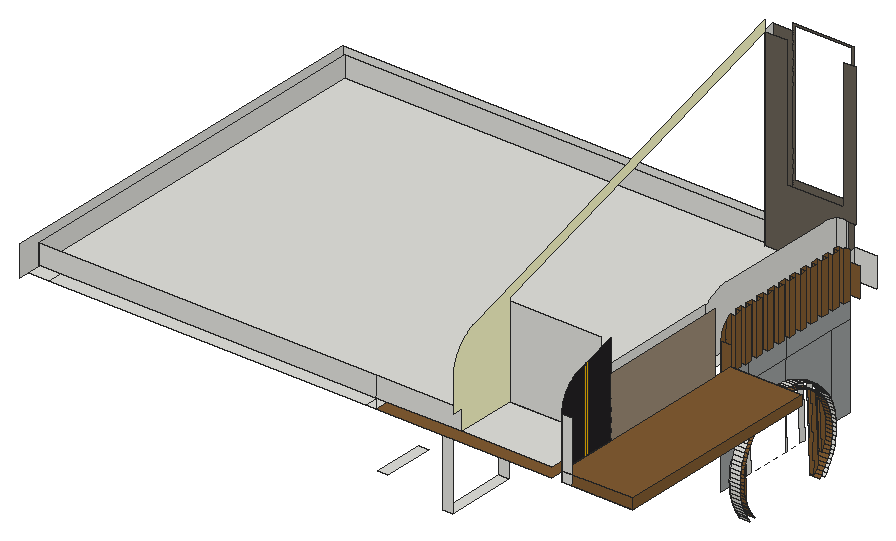
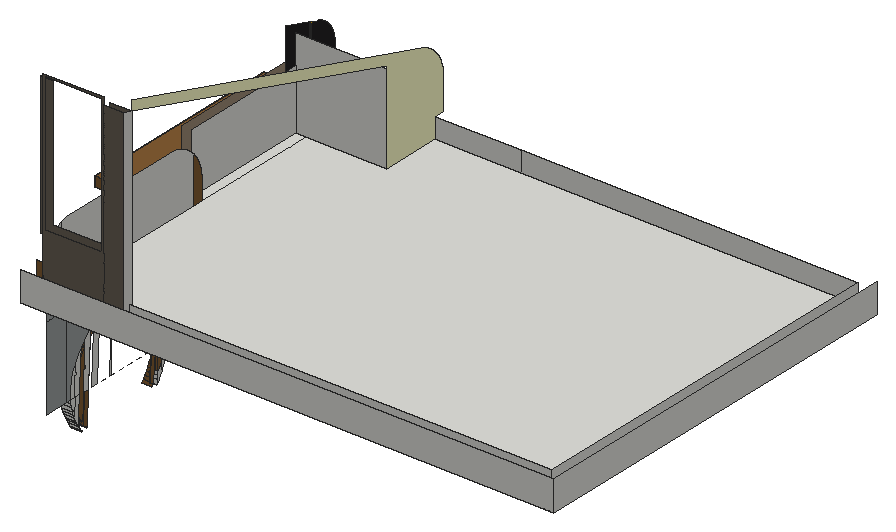
# SketchUp Ruby script. Lengths in inches.
U = 1.inch
M = Sketchup.active_model
def pt(a) = Geom::Point3d.new(a.map { |v| v * U })
def face(e, loops, mat)
  f = e.add_face(loops[0].map { |a| pt(a) })
  loops[1..].each { |l| e.add_face(l.map { |a| pt(a) }).erase! }
  f.material = f.back_material = mat if mat
  f
end
# faces: each face lists its corners as indices into pts; further lists are holes
def faces(e, pts, list, mat = nil) = list.each { |f| face(e, (f[0].is_a?(Array) ? f : [f]).map { |l| l.map { |i| pts[i] } }, mat) }
# xy, xz, yz: faces in a plane at the given z, y or x. An outline is a flat list of corners, or four numbers for a rectangle; further outlines are holes
def ring(l) = l.size == 4 ? [[l[0], l[1]], [l[2], l[1]], [l[2], l[3]], [l[0], l[3]]] : l.each_slice(2).to_a
def flat(e, list, mat, &to3) = list.each { |f| face(e, (f[0].is_a?(Array) ? f : [f]).map { |l| ring(l).map { |u, v| to3.(u, v) } }, mat) }
def xy(e, z, list, mat = nil) = flat(e, list, mat) { |x, y| [x, y, z] }
def xz(e, y, list, mat = nil) = flat(e, list, mat) { |x, z| [x, y, z] }
def yz(e, x, list, mat = nil) = flat(e, list, mat) { |y, z| [x, y, z] }
def lines(e, pts, list) = list.each { |a, b| e.add_line(pt(pts[a]), pt(pts[b])) }
# prism: a flat outline (further loops are holes) pulled along v
def prism(e, loops, v, mat = nil)
  f = face(e, loops, mat); d = Geom::Vector3d.new(v.map { |x| x * U })
  f.pushpull(f.normal.samedirection?(d) ? d.length : -d.length)
end
def box(e, o, s, mat = nil) = prism(e, [[o, [o[0] + s[0], o[1], o[2]], [o[0] + s[0], o[1] + s[1], o[2]], [o[0], o[1] + s[1], o[2]]]], [0, 0, s[2]], mat)
def at(x, y, z, deg = 0) = Geom::Transformation.translation(pt([x, y, z])) * Geom::Transformation.rotation(ORIGIN, Z_AXIS, deg.degrees)
def axes(o, x, y, z) = Geom::Transformation.new([*x, 0, *y, 0, *z, 0, *pt(o).to_a, 1])
def part(name) = M.definitions.add(name)
# library, detail: a bought-in or finely detailed component or shape, given as its bounding box
def library(name, o, s) = part(name).tap { |d| box(d.entities, o, s) }
def detail(e, o, s) = box(e.add_group.entities, o, s)
def put(e, d, t, mat = nil) = e.add_instance(d, t).tap { |i| i.material = mat if mat }
def group(e, t, mat = nil) = e.add_group.tap { |g| g.transformation = t; g.material = mat if mat }.entities
root = M.entities
M.materials.add("C08_Toffee_Ember").color = [130, 92, 50]
M.materials.add("D05_Goldenrod_Hue").color = [255, 191, 0]
M.materials.add("Denim_03_1K").color = [156, 160, 160]
M.materials.add("E01_Mint_Frost").color = [255, 255, 204]
M.materials.add("Marble_07_1K").color = [36, 34, 36]
M.materials.add("Plaster_02_1K").color = [157, 140, 119]
M.materials.add("Plaster_04_1K").color = [106, 98, 87]
xy(root,297,[[206.67,78,212.67,120]])
xy(root,339,[[206.67,30,212.67,60],[206.67,78,212.67,120]])
xy(root,378,[[5.5,21,17.5,141],[17.5,21,206.67,141],[206.67,21,212.67,141],[212.67,135,311.5,141],[5.5,141,17.5,255],
  [17.5,141,311.5,249],[317.5,154.16,320.5,157.74],[317.5,161.32,320.5,165.4],[317.5,169.49,320.5,173.57],[317.5,177.66,320.5,181.74],
  [317.5,185.82,320.5,189.91],[317.5,193.99,320.5,198.08],[317.5,202.16,320.5,206.24],[317.5,210.33,320.5,214.41],[317.5,218.5,320.5,222.58],
  [317.5,226.66,320.5,230.75],[317.5,234.83,320.5,238.92]])
xy(root,378,[[212.67,21,212.67,135,329.5,135,329.5,147,365.5,147,365.5,21,323.5,21,323.5,57,317.5,57,317.5,21]],"C08_Toffee_Ember")
xy(root,382.3,[[263.5,247,311.5,253]])
xy(root,384,[[11.5,21,263.5,21,263.5,57,311.5,57,311.5,249,11.5,249],[263.5,21,317.5,57],[311.5,57,317.5,135]])
xy(root,384,[[323.5,21,365.5,147]],"C08_Toffee_Ember")
xz(root,21,[[323.5,378,329.5,384],[11.5,384,212.67,396],[212.67,384,263.5,396],[323.5,384,329.5,414]])
xz(root,21,[[329.5,378,365.5,384]],"C08_Toffee_Ember")
xz(root,57,[[263.5,384,317.5,437.47]])
xz(root,78,[[206.67,297,212.67,339]])
xz(root,120,[[206.67,297,212.67,339]])
xz(root,135,[[311.5,384,317.5,396],[317.5,384,323.5,396]])
xz(root,147,[[317.5,378,317.5,396,323.5,396,323.5,384,365.5,384,365.5,378]],"C08_Toffee_Ember")
xz(root,154.16,[[317.5,378,320.5,406.92]],"C08_Toffee_Ember")
xz(root,157.74,[[317.5,378,320.5,407.92]],"C08_Toffee_Ember")
xz(root,161.32,[[317.5,378,320.5,408]],"C08_Toffee_Ember")
xz(root,165.4,[[317.5,378,320.5,408]],"C08_Toffee_Ember")
xz(root,169.49,[[317.5,378,320.5,408]],"C08_Toffee_Ember")
xz(root,173.57,[[317.5,378,320.5,408]],"C08_Toffee_Ember")
xz(root,177.66,[[317.5,378,320.5,408]],"C08_Toffee_Ember")
xz(root,181.74,[[317.5,378,320.5,408]],"C08_Toffee_Ember")
xz(root,185.82,[[317.5,378,320.5,408]],"C08_Toffee_Ember")
xz(root,189.91,[[317.5,378,320.5,408]],"C08_Toffee_Ember")
xz(root,193.99,[[317.5,378,320.5,408]],"C08_Toffee_Ember")
xz(root,198.08,[[317.5,378,320.5,408]],"C08_Toffee_Ember")
xz(root,202.16,[[317.5,378,320.5,408]],"C08_Toffee_Ember")
xz(root,206.24,[[317.5,378,320.5,408]],"C08_Toffee_Ember")
xz(root,210.33,[[317.5,378,320.5,408]],"C08_Toffee_Ember")
xz(root,214.41,[[317.5,378,320.5,408]],"C08_Toffee_Ember")
xz(root,218.5,[[317.5,378,320.5,408]],"C08_Toffee_Ember")
xz(root,222.58,[[317.5,378,320.5,408]],"C08_Toffee_Ember")
xz(root,226.66,[[317.5,378,320.5,408]],"C08_Toffee_Ember")
xz(root,230.75,[[317.5,378,320.5,408]],"C08_Toffee_Ember")
xz(root,234.83,[[317.5,378,320.5,407.41]],"C08_Toffee_Ember")
xz(root,238.92,[[317.5,378,320.5,405.09]],"C08_Toffee_Ember")
xz(root,243,[[317.5,378,323.5,396]],"C08_Toffee_Ember")
xz(root,247,[[263.5,382.3,311.5,382.3,311.5,413.98,317.5,413.98,317.5,498,310.5,498,310.5,421,276.5,421,276.5,498,263.5,498]],"Plaster_04_1K")
xz(root,249,[[11.5,384,311.5,396]])
xz(root,253,[[263.5,382.3,275.5,500.01],[275.5,382.3,275.5,500.01,276.5,500.01,276.5,421,310.5,421,310.5,503,276.5,503,276.5,500.01,275.5,500.01,275.5,504,311.5,504,311.5,382.3]],"Plaster_04_1K")
xz(root,255,[[5.5,378,323.5,396]])
yz(root,5.5,[[15,378,255,396]])
yz(root,11.5,[[21,384,249,396]])
yz(root,263.5,[[247,382.3,247,498.15,253,500.01,253,382.3]])
yz(root,263.5,[[21,384,21,396,15,396,15,415.29,15.02,415.87,15.0625,416.5,15.12,417.12,15.19,417.74,15.28,418.36,15.39,418.97,15.51,419.58,15.65,420.19,15.81,420.8,15.98,421.4,16.16,421.99,16.58,423.17,16.82,423.75,17.07,424.32,17.33,424.89,17.61,425.44,17.9,426,18.21,426.54,18.53,427.07,18.87,427.6,19.22,428.12,19.58,428.625,19.96,429.12,20.35,429.61,20.75,430.09,21,430.37,21.17,430.55,21.59,431.01,22.03,431.45,22.49,431.88,22.61,432,22.95,432.3,23.42,432.71,23.9,433.1,24.4,433.49,24.9,433.85,25.42,434.21,25.9375,434.55,26.47,434.88,27.01,435.19,27.56,435.49,28.12,435.77,28.68,436.04,29.25,436.3,29.83,436.54,30.41,436.76,30.96,436.95,247,504,247,498,57,439.04,57,384]],"E01_Mint_Frost")
yz(root,311.5,[[247,382.3,253,382.3,253,396,249,396,249,384,247,384],[141,384,141,411.58,141.14,411.74,141.65,412.29,142.17,412.83,142.71,413.35,143.26,413.86,143.83,414.35,144.41,414.82,145.01,415.27,145.625,415.7,146.25,416.12,146.89,416.52,147.53,416.89,148.19,417.25,148.86,417.58,149.55,417.9,150.24,418.19,150.93,418.46,151.64,418.71,152.35,418.94,153.08,419.15,153.8,419.34,154.53,419.5,155.27,419.64,156.01,419.76,156.76,419.85,157.5,419.92,158.25,419.97,159,420,231,420,231.76,419.99,232.51,419.96,233.26,419.91,234.01,419.83,234.76,419.73,235.51,419.6,236.25,419.45,236.98,419.28,237.71,419.08,238.4375,418.86,239.15,418.62,239.59,418.46,239.59,384],[239.59,384,239.59,418.46,239.86,418.36,240.56,418.07,241.25,417.76,241.93,417.43,242.6,417.08,243.25,416.71,243.9,416.3125,244.53,415.9,245.15,415.47,245.75,415.01,246.34,414.54,246.92,414.05,247,413.98,247,384],[247,384,249,384,249,411.97,248.54,412.48,248.02,413.02,247.48,413.54,247,413.98]])
yz(root,311.5,[[135,384,135,396,135.03,396.75,135.08,397.5,135.15,398.24,135.24,398.99,135.36,399.73,135.5,400.47,135.66,401.2,135.85,401.92,136.06,402.65,136.29,403.36,136.54,404.07,136.81,404.76,137.1,405.45,137.42,406.14,137.75,406.81,138.11,407.47,138.48,408.11,138.88,408.75,139.3,409.375,139.73,409.99,140.18,410.59,140.65,411.17,141,411.58,141,384]],"C08_Toffee_Ember")
yz(root,317.5,[[160.39,296.18,160.08,302.125,159.9,302.43,158.98,304.29,158.18,306.2,157.5,308.16,156.95,310.15,156.52,312.18,156.22,314.23,156.125,315.33,156.09,315.33,156.78,301.98,157.26,301.01,158.39,299.05,159.64,297.17],[219.71,299.24,220.35,300.3,221.4,302.31,222.32,304.37,222.7,305.375,222.18,315.33,218.88,315.33,219.4,305.1875],[156.78,301.98,156.09,315.33,153.12,315.33,153.24,313.89,153.5625,311.65,154.03,309.44,154.64,307.26,155.38,305.125,156.26,303.04],[222.7,305.375,223.11,306.49,223.77,308.65,224.28,310.86,224.66,313.09,224.9,315.33,222.18,315.33],[153.12,315.33,156.09,315.33,156.04,316.3,155.3,330.625,154.89,329.51,154.23,327.35,153.72,325.14,153.34,322.91,153.1,320.67,153,318.41,153.05,316.14],
  [156.09,315.33,156.125,315.33,156.04,316.3],[159.4,315.33,162.7,315.33,161.62,336.39,161.375,341.07,160.12,339.49,158.82,337.63,158.29,336.76,158.6,330.8125],[166.01,315.33,169.3125,315.33,167.87,343.33,167.68,346.99,166.37,346,164.65,344.52,164.51,344.375,164.72,340.32],[194.92,315.33,195.75,315.33,194.92,331.43],[205.66,315.33,208.96,315.33,207.41,345.37,207.23,349.03,206.7,349.35,204.69,350.4,203.83,350.78,204.01,347.375],
  [212.27,315.33,215.57,315.33,214.35,339.11,214.1,343.79,213.9375,343.96,212.26,345.48,210.65,346.76,210.86,342.71],[218.88,315.33,222.18,315.33,221.96,319.7,221.22,334.02,220.74,334.99,219.61,336.95,218.36,338.83,217.61,339.82,217.92,333.875],[222.18,315.33,224.9,315.33,225,317.59,224.95,319.86,224.76,322.11,224.4375,324.35,223.97,326.56,223.36,328.74,222.62,330.875,221.74,332.96,221.22,334.02,221.96,319.7],[57,384,135,420]])
yz(root,317.5,[[216.38,299.61,216.66,300,217.74,301.78,218.7,303.61,219.4,305.1875,218.88,315.33,217.92,333.875,217.0625,335.37,215.91,337.09,214.66,338.75,214.35,339.11,215.57,315.33],[160.08,302.125,159.4,315.33,158.6,330.8125,158.46,330.49,157.73,328.55,157.13,326.57,156.66,324.55,156.31,322.51,156.09,320.44,156,318.37,156.04,316.3,156.125,315.33,156.22,314.23,156.52,312.18,156.95,310.15,157.5,308.16,158.18,306.2,158.98,304.29,159.9,302.43],[194.92,331.43,194.92,350.45,193.93,350.62],[147,378,150.58,378,150.58,404.46,150.56,404.44,150.3,404.17,149.8,403.61,149.57,403.3125,149.34,403.01,149.12,402.71,148.72,402.07,148.53,401.75,148.35,401.42,148.1875,401.08,148.03,400.74,147.88,400.39,147.75,400.04,147.625,399.6875,147.51,399.33,147.41,398.97,147.32,398.61,147.24,398.24,147.17,397.87,147.11,397.5,147.03,396.75,147.01,396.375,147,396],[150.58,378,154.16,378,154.16,406.92,153.92,406.8125,153.58,406.65,153.25,406.47,152.93,406.28,152.29,405.88,151.99,405.66,151.6875,405.43,151.39,405.2,150.83,404.7,150.58,404.46],
  [157.74,378,161.32,378,161.32,408,159,408,158.625,407.99,158.25,407.97,157.875,407.93,157.74,407.92],[165.4,378,169.49,408],[173.57,378,177.66,408],[181.74,378,185.82,408],[189.91,378,193.99,408],
  [198.08,378,202.16,408],[206.24,378,210.33,408],[214.41,378,218.5,408],[222.58,378,226.66,408],[230.75,378,234.83,378,234.83,407.41,234.72,407.45,234,407.65,233.63,407.74,233.26,407.81,232.88,407.87,232.51,407.92,232.13,407.96,231.76,407.98,231.38,408,230.75,408],
  [238.92,378,243,378,243,396.38,242.98,396.76,242.96,397.13,242.92,397.51,242.87,397.88,242.81,398.26,242.74,398.63,242.65,399,242.45,399.72,242.33,400.08,242.19,400.4375,242.05,400.79,241.9,401.13,241.56,401.81,241.37,402.14,240.97,402.78,240.75,403.09,240.52,403.39,240.29,403.6875,240.04,403.97,239.79,404.25,239.53,404.53,239.25,404.79,238.97,405.04,238.92,405.09]],"C08_Toffee_Ember")
yz(root,317.5,[[147,315.33,153.12,315.33,153.05,316.14,153,318.41,153.1,320.67,153.34,322.91,153.72,325.14,154.23,327.35,154.89,329.51,155.3,330.625,155.68,331.63,156.6,333.69,157.65,335.7,158.29,336.76,158.82,337.63,160.12,339.49,161.375,341.07,161.52,341.26,163.04,342.9375,164.51,344.375,164.65,344.52,166.37,346,167.68,346.99,167.68,365.07,147,365.07],[224.9,315.33,228.75,315.33,228.75,365.07,194.92,365.07,194.92,353.49,196.14,353.28,198.35,352.77,200.51,352.11,202.63,351.32,203.83,350.78,204.69,350.4,206.7,349.35,207.23,349.03,208.63,348.18,210.49,346.88,210.65,346.76,212.26,345.48,213.9375,343.96,214.1,343.79,215.52,342.35,217,340.63,217.61,339.82,218.36,338.83,219.61,336.95,220.74,334.99,221.22,334.02,221.74,332.96,222.62,330.875,223.36,328.74,223.97,326.56,224.4375,324.35,224.76,322.11,224.95,319.86,225,317.59],[228.75,315.33,243,365.07],[167.68,346.99,168.17,347.36,170.05,348.61,170.875,349.08,172.01,349.74,174.04,350.74,176.125,351.62,178.26,352.36,180.44,352.97,182.65,353.4375,184.89,353.76,187.14,353.95,189.41,354,191.67,353.9,193.91,353.66,194.92,353.49,194.92,365.07,167.68,365.07],[147,365.07,167.68,378],
  [167.68,365.07,194.92,378],[194.92,365.07,243,378]],"Denim_03_1K")
yz(root,319.5,[[213.28,295.68,214.1875,296.68,215.48,298.3,216.38,299.61,214.35,339.11,213.31,340.32,211.86,341.8,210.86,342.71],[163.65,296.89,161.62,336.39,161.34,336,160.26,334.22,159.3,332.39,158.6,330.8125,160.08,302.125,160.9375,300.63,162.09,298.91,163.34,297.25],[219.4,305.1875,219.54,305.51,220.27,307.45,220.87,309.43,221.34,311.45,221.69,313.49,221.91,315.56,222,317.63,221.96,319.7,221.78,321.77,221.48,323.82,221.05,325.85,220.5,327.84,219.82,329.8,219.02,331.71,218.1,333.57,217.92,333.875]],"C08_Toffee_Ember")
yz(root,320.5,[[154.16,378,157.74,378,157.74,407.92,157.5,407.89,157.13,407.83,156.76,407.76,156.39,407.68,156.03,407.59,155.67,407.49,155.3125,407.375,154.96,407.25,154.61,407.12,154.26,406.97,154.16,406.92],[161.32,378,165.4,408],[169.49,378,173.57,408],[177.66,378,181.74,408],[185.82,378,189.91,408],
  [193.99,378,198.08,408],[202.16,378,206.24,408],[210.33,378,214.41,408],[218.5,378,222.58,408],[226.66,378,230.75,408],
  [234.83,378,238.92,378,238.92,405.09,238.6875,405.29,238.39,405.52,238.09,405.75,237.78,405.97,237.14,406.37,236.81,406.56,236.13,406.9,235.79,407.05,235.4375,407.19,235.08,407.33,234.83,407.41]],"C08_Toffee_Ember")
yz(root,323.5,[[21,378,38,384],[38,378,39,384],[39,378,40,384],[40,378,57,384]])
yz(root,323.5,[[38,384,39,384,39,433.45,38,433.14],[39,384,40,384,40,433.76,39,433.45]],"D05_Goldenrod_Hue")
yz(root,323.5,[[21,384,38,384,38,433.14,33.4375,431.72,32.99,431.57,32.54,431.41,32.1,431.23,31.67,431.05,31.23,430.85,30.81,430.64,30.39,430.42,29.98,430.1875,29.57,429.94,29.17,429.69,28.77,429.43,28.01,428.87,27.63,428.58,26.91,427.96,26.57,427.64,26.23,427.3,25.9,426.96,25.26,426.26,24.96,425.89,24.67,425.52,24.39,425.14,24.11,424.75,23.85,424.35,23.6,423.95,23.36,423.54,23.13,423.13,22.91,422.71,22.7,422.28,22.51,421.85,22.32,421.41,22.15,420.97,21.99,420.53,21.84,420.08,21.7,419.625,21.57,419.17,21.46,418.71,21.36,418.24,21.27,417.78,21.19,417.31,21.125,416.84,21.07,416.37,21.03,415.9,21.01,415.42,21,415.2],[40,384,57,384,57,439.04,40,433.76]],"Marble_07_1K")
yz(root,323.5,[[57,384,135,420]],"Plaster_02_1K")
yz(root,365.5,[[21,378,147,384]],"C08_Toffee_Ember")
p = [[317.5,216.625,294.93],[317.5,217.88,296.51],[323.5,217.88,296.51],[323.5,216.48,294.74],[317.5,216.48,294.74],[323.5,214.1875,296.68],
  [319.5,214.1875,296.68],[319.5,213.28,295.68],[317.5,213.28,295.68],[317.5,212.8,295.14],[323.5,212.8,295.14],[317.5,160.39,296.18],
  [317.5,161,295.37],[323.5,161,295.37],[323.5,159.64,297.17],[317.5,159.64,297.17],[317.5,164.69,295.68],[317.5,163.65,296.89],
  [319.5,163.65,296.89],[319.5,163.34,297.25],[323.5,163.34,297.25],[323.5,164.69,295.68],[317.5,210.86,342.71],[317.5,212.27,315.33],
  [319.5,210.86,342.71],[317.5,219.18,298.37],[323.5,219.18,298.37],[323.5,215.48,298.3],[319.5,215.48,298.3],[317.5,162.7,315.33],
  [317.5,161.62,336.39],[319.5,161.62,336.39],[317.5,158.39,299.05],[323.5,158.39,299.05],[319.5,162.09,298.91],[323.5,162.09,298.91],
  [323.5,216.66,300],[317.5,216.66,300],[317.5,216.38,299.61],[319.5,216.38,299.61],[317.5,219.71,299.24],[317.5,220.35,300.3],
  [323.5,220.35,300.3],[319.5,160.9375,300.63],[323.5,160.9375,300.63],[317.5,157.26,301.01],[323.5,157.26,301.01],[319.5,214.35,339.11],
  [317.5,215.57,315.33],[317.5,214.35,339.11],[323.5,217.74,301.78],[317.5,217.74,301.78],[317.5,221.4,302.31],[323.5,221.4,302.31],
  [319.5,160.08,302.125],[317.5,160.08,302.125],[317.5,159.9,302.43],[323.5,159.9,302.43],[317.5,156.78,301.98],[323.5,156.26,303.04],
  [317.5,156.26,303.04],[323.5,218.7,303.61],[317.5,218.7,303.61],[317.5,158.6,330.8125],[317.5,159.4,315.33],[319.5,158.6,330.8125],
  [317.5,222.32,304.37],[323.5,222.32,304.37],[317.5,158.98,304.29],[323.5,158.98,304.29],[317.5,155.38,305.125],[323.5,155.38,305.125],
  [323.5,219.54,305.51],[319.5,219.54,305.51],[319.5,219.4,305.1875],[317.5,219.4,305.1875],[317.5,158.18,306.2],[323.5,158.18,306.2],
  [317.5,222.7,305.375],[317.5,223.11,306.49],[323.5,223.11,306.49],[317.5,154.64,307.26],[323.5,154.64,307.26],[317.5,217.92,333.875],
  [317.5,218.88,315.33],[319.5,217.92,333.875],[323.5,220.27,307.45],[319.5,220.27,307.45],[317.5,157.5,308.16],[323.5,157.5,308.16],
  [317.5,223.77,308.65],[323.5,223.77,308.65],[317.5,154.03,309.44],[323.5,154.03,309.44],[323.5,220.87,309.43],[319.5,220.87,309.43],
  [317.5,156.95,310.15],[323.5,156.95,310.15],[317.5,224.28,310.86],[323.5,224.28,310.86],[317.5,153.5625,311.65],[323.5,153.5625,311.65],
  [323.5,221.34,311.45],[319.5,221.34,311.45],[317.5,156.52,312.18],[323.5,156.52,312.18],[317.5,224.66,313.09],[323.5,224.66,313.09],
  [323.5,221.69,313.49],[319.5,221.69,313.49],[317.5,153.24,313.89],[323.5,153.24,313.89],[317.5,156.22,314.23],[323.5,156.22,314.23],
  [317.5,224.9,315.33],[323.5,224.9,315.33],[323.5,221.91,315.56],[319.5,221.91,315.56],[317.5,153.12,315.33],[323.5,153.05,316.14],
  [317.5,153.05,316.14],[317.5,156.125,315.33],[317.5,156.04,316.3],[323.5,156.04,316.3],[317.5,225,317.59],[323.5,225,317.59],
  [323.5,222,317.63],[319.5,222,317.63],[317.5,153,318.41],[323.5,153,318.41],[317.5,156,318.37],[323.5,156,318.37],
  [323.5,221.96,319.7],[319.5,221.96,319.7],[317.5,224.95,319.86],[323.5,224.95,319.86],[317.5,153.1,320.67],[323.5,153.1,320.67],
  [317.5,156.09,320.44],[323.5,156.09,320.44],[323.5,221.78,321.77],[319.5,221.78,321.77],[317.5,224.76,322.11],[323.5,224.76,322.11],
  [317.5,156.31,322.51],[323.5,156.31,322.51],[317.5,153.34,322.91],[323.5,153.34,322.91],[323.5,221.48,323.82],[319.5,221.48,323.82],
  [317.5,224.4375,324.35],[323.5,224.4375,324.35],[317.5,156.66,324.55],[323.5,156.66,324.55],[317.5,153.72,325.14],[323.5,153.72,325.14],
  [323.5,221.05,325.85],[319.5,221.05,325.85],[317.5,223.97,326.56],[323.5,223.97,326.56],[317.5,157.13,326.57],[323.5,157.13,326.57],
  [317.5,154.23,327.35],[323.5,154.23,327.35],[323.5,220.5,327.84],[319.5,220.5,327.84],[317.5,157.73,328.55],[323.5,157.73,328.55],
  [317.5,223.36,328.74],[323.5,223.36,328.74],[317.5,154.89,329.51],[323.5,154.89,329.51],[323.5,219.82,329.8],[319.5,219.82,329.8],
  [317.5,158.46,330.49],[323.5,158.46,330.49],[317.5,222.62,330.875],[323.5,222.62,330.875],[317.5,155.3,330.625],[323.5,155.68,331.63],
  [317.5,155.68,331.63],[323.5,219.02,331.71],[319.5,219.02,331.71],[319.5,159.3,332.39],[323.5,159.3,332.39],[317.5,221.74,332.96],
  [323.5,221.74,332.96],[317.5,156.6,333.69],[323.5,156.6,333.69],[323.5,218.1,333.57],[319.5,218.1,333.57],[319.5,160.26,334.22],
  [323.5,160.26,334.22],[317.5,221.22,334.02],[317.5,220.74,334.99],[323.5,220.74,334.99],[323.5,217.0625,335.37],[317.5,217.0625,335.37],
  [317.5,157.65,335.7],[323.5,157.65,335.7],[319.5,161.34,336],[323.5,161.34,336],[317.5,219.61,336.95],[323.5,219.61,336.95],
  [323.5,215.91,337.09],[317.5,215.91,337.09],[317.5,158.29,336.76],[323.5,158.82,337.63],[317.5,158.82,337.63],[317.5,162.52,337.7],
  [323.5,162.52,337.7],[317.5,218.36,338.83],[323.5,218.36,338.83],[323.5,214.66,338.75],[317.5,214.66,338.75],[317.5,160.12,339.49],
  [323.5,160.12,339.49],[317.5,163.8125,339.32],[323.5,163.8125,339.32],[323.5,213.31,340.32],[319.5,213.31,340.32],[317.5,217.61,339.82],
  [317.5,217,340.63],[323.5,217,340.63],[317.5,164.72,340.32],[319.5,164.72,340.32],[319.5,165.2,340.86],[323.5,165.2,340.86],
  [317.5,161.375,341.07],[323.5,161.52,341.26],[317.5,161.52,341.26],[323.5,211.86,341.8],[319.5,211.86,341.8],[317.5,215.52,342.35],
  [323.5,215.52,342.35],[319.5,166.68,342.31],[323.5,166.68,342.31],[317.5,163.04,342.9375],[323.5,163.04,342.9375],[317.5,210.32,343.1875],
  [323.5,210.32,343.1875],[319.5,167.87,343.33],[317.5,167.87,343.33],[317.5,168.25,343.66],[323.5,168.25,343.66],[317.5,214.1,343.79],
  [317.5,213.9375,343.96],[323.5,213.9375,343.96],[317.5,164.51,344.375],[323.5,164.65,344.52],[317.5,164.65,344.52],[317.5,208.7,344.48],
  [323.5,208.7,344.48],[317.5,169.91,344.91],[323.5,169.91,344.91],[317.5,212.26,345.48],[323.5,212.26,345.48],[317.5,166.37,346],
  [323.5,166.37,346],[323.5,207,345.66],[319.5,207,345.66],[319.5,207.41,345.37],[317.5,207.41,345.37],[317.5,171.05,345.67],
  [319.5,171.05,345.67],[319.5,171.63,346.0625],[323.5,171.63,346.0625],[317.5,210.65,346.76],[317.5,210.49,346.88],[323.5,210.49,346.88],
  [323.5,205.22,346.74],[319.5,205.22,346.74],[317.5,167.68,346.99],[323.5,168.17,347.36],[317.5,168.17,347.36],[319.5,173.43,347.1],
  [323.5,173.43,347.1],[317.5,203.39,347.7],[317.5,204.01,347.375],[319.5,204.01,347.375],[323.5,203.39,347.7],[317.5,208.63,348.18],
  [323.5,208.63,348.18],[319.5,174.26,347.51],[317.5,174.26,347.51],[317.5,175.29,348.02],[323.5,175.29,348.02],[317.5,170.05,348.61],
  [323.5,170.05,348.61],[317.5,201.49,348.54],[323.5,201.49,348.54],[317.5,177.2,348.82],[323.5,177.2,348.82],[317.5,207.23,349.03],
  [317.5,206.7,349.35],[323.5,206.7,349.35],[323.5,199.55,349.27],[319.5,199.55,349.27],[319.5,200.625,348.87],[317.5,200.625,348.87],
  [317.5,170.875,349.08],[323.5,172.01,349.74],[317.5,172.01,349.74],[317.5,177.49,348.92],[319.5,177.49,348.92],[319.5,179.16,349.5],
  [323.5,179.16,349.5],[323.5,197.57,349.87],[319.5,197.57,349.87],[317.5,204.69,350.4],[323.5,204.69,350.4],[319.5,180.74,349.9375],
  [317.5,180.74,349.9375],[317.5,181.15,350.05],[323.5,181.15,350.05],[317.5,174.04,350.74],[323.5,174.04,350.74],[317.5,195.55,350.34],
  [317.5,197.27,349.94],[319.5,197.27,349.94],[323.5,195.55,350.34],[317.5,183.18,350.48],[323.5,183.18,350.48],[323.5,193.51,350.69],
  [319.5,193.51,350.69],[319.5,193.93,350.62],[317.5,193.93,350.62],[317.5,194.92,350.45],[317.5,203.83,350.78],[317.5,202.63,351.32],
  [323.5,202.63,351.32],[317.5,184.01,350.61],[319.5,184.01,350.61],[319.5,185.23,350.78],[323.5,185.23,350.78],[317.5,176.125,351.62],
  [323.5,176.125,351.62],[323.5,191.44,350.91],[319.5,191.44,350.91],[319.5,187.3,350.96],[323.5,187.3,350.96],[317.5,189.37,351],
  [317.5,190.6,350.95],[319.5,190.6,350.95],[323.5,189.37,351],[317.5,187.3,350.96],[317.5,200.51,352.11],[323.5,200.51,352.11],
  [317.5,178.26,352.36],[323.5,178.26,352.36],[317.5,198.35,352.77],[323.5,198.35,352.77],[317.5,180.44,352.97],[323.5,180.44,352.97],
  [317.5,196.14,353.28],[323.5,196.14,353.28],[317.5,182.65,353.4375],[323.5,182.65,353.4375],[317.5,194.92,353.49],[317.5,193.91,353.66],
  [323.5,193.91,353.66],[317.5,184.89,353.76],[323.5,184.89,353.76],[317.5,191.67,353.9],[323.5,191.67,353.9],[317.5,187.14,353.95],
  [323.5,187.14,353.95],[317.5,189.41,354],[323.5,189.41,354],[212.67,21,378],[212.67,21,384],[317.5,221.96,319.7],
  [317.5,190.6,351.125],[317.5,193.89,351.3],[317.5,197.1875,351.47],[317.5,200.48,351.64],[317.5,184,350.79],[317.5,180.71,350.62],
  [317.5,177.41,350.45],[317.5,174.12,350.28],[317.5,146.83,378],[317.5,147,378],[317.5,194.92,315.33],[317.5,192.44,315.33],
  [317.5,189.14,315.33],[317.5,185.83,315.33],[317.5,202.36,315.33],[317.5,199.05,315.33],[317.5,175.92,315.33],[317.5,172.62,315.33],
  [317.5,182.53,315.33],[317.5,179.22,315.33]]
faces(root,p,[[0,1,2,3,4],[11,12,13,14,15],[1,25,26,2],[32,15,14,33],[40,41,42,26,25],[45,32,33,46],[41,52,53,42],[58,45,46,59,60],
  [52,66,67,53],[70,60,59,71],[78,79,80,67,66],[81,70,71,82],[79,90,91,80],[92,81,82,93],[90,98,99,91],[100,92,93,101],
  [98,106,107,99],[110,100,101,111],[106,114,115,107],[118,110,111,119,120],[114,124,125,115],[128,120,119,129],[124,134,135,125],[136,128,129,137],
  [134,142,143,135],[146,136,137,147],[142,150,151,143],[154,146,147,155],[150,158,159,151],[162,154,155,163],[158,168,169,159],[170,162,163,171],
  [168,176,177,169],[178,170,171,179,180],[176,185,186,177],[187,180,179,188],[193,194,195,186,185],[198,187,188,199],[194,202,203,195],[206,198,199,207,208],
  [202,211,212,203],[215,208,207,216],[221,222,223,212,211],[228,215,216,229,230],[222,233,234,223],[237,230,229,238],[245,246,247,234,233],[248,237,238,249,250],
  [246,255,256,247],[257,250,249,258],[267,268,269,256,255],[272,257,258,273,274],[268,281,282,269],[287,274,273,288],[293,294,295,282,281],[300,287,288,301,302],
  [294,309,310,295],[315,302,301,316],[328,329,330,310,309],[335,315,316,336],[329,346,347,330],[348,335,336,349],[346,350,351,347],[352,348,349,353],
  [350,354,355,351],[356,352,353,357],[358,359,360,355,354],[361,356,357,362],[359,363,364,360],[365,361,362,366],[363,367,368,364],[367,365,366,368]])
faces(root,p,[[5,6,7,8,9,10],[16,17,18,19,20,21],[22,23,8,7,24],[27,28,6,5],[29,30,31,18,17],[20,19,34,35],[36,37,38,39,28,27],[35,34,43,44],
  [47,39,38,48,49],[50,51,37,36],[44,43,54,55,56,57],[61,62,51,50],[63,64,55,54,65],[56,68,69,57],[72,73,74,75,62,61],[68,76,77,69],
  [83,84,75,74,85],[86,87,73,72],[76,88,89,77],[94,95,87,86],[88,96,97,89],[102,103,95,94],[96,104,105,97],[108,109,103,102],
  [104,112,113,105],[116,117,109,108],[112,121,122,123,113],[126,127,117,116],[122,130,131,123],[132,133,127,126],[130,138,139,131],[140,141,133,132],
  [138,144,145,139],[148,149,141,140],[144,152,153,145],[156,157,149,148],[152,160,161,153],[164,165,157,156],[160,166,167,161],[172,173,165,164],
  [166,174,175,167],[181,182,173,172],[174,63,65,183,184,175],[189,190,182,181],[184,183,191,192],[196,197,83,85,190,189],[192,191,200,201],[204,205,197,196],
  [201,200,31,30,209,210],[213,214,205,204],[209,217,218,210],[219,220,47,49,214,213],[217,224,225,226,227,218],[231,232,220,219],[227,226,235,236],[239,22,24,232,231,240],
  [236,235,241,242,243,244],[251,239,240,252],[243,253,254,244],[259,260,261,262,251,252],[253,263,264,265,266,254],[270,271,260,259],[266,265,275,276],[277,278,279,271,270,280],
  [276,275,283,284,285,286],[289,277,280,290],[285,291,292,286],[296,297,298,299,289,290],[291,303,304,305,306,292],[307,308,297,296],[306,305,311,312,313,314],[317,318,319,308,307,320],
  [313,321,322,314],[323,324,325,326,327,317,320],[321,331,332,333,334,322],[337,338,324,323],[334,333,339,340],[341,342,343,338,337,344],[345,341,344,340,339]],"C08_Toffee_Ember")
lines(root,p,[[369,370],[133,371],[372,342],[373,326],[374,318],[375,299],[376,331],[377,312],[378,303],[379,284],[300,263],[327,358],
  [380,381],[382,383],[384,385],[386,387],[388,389],[390,391]])
